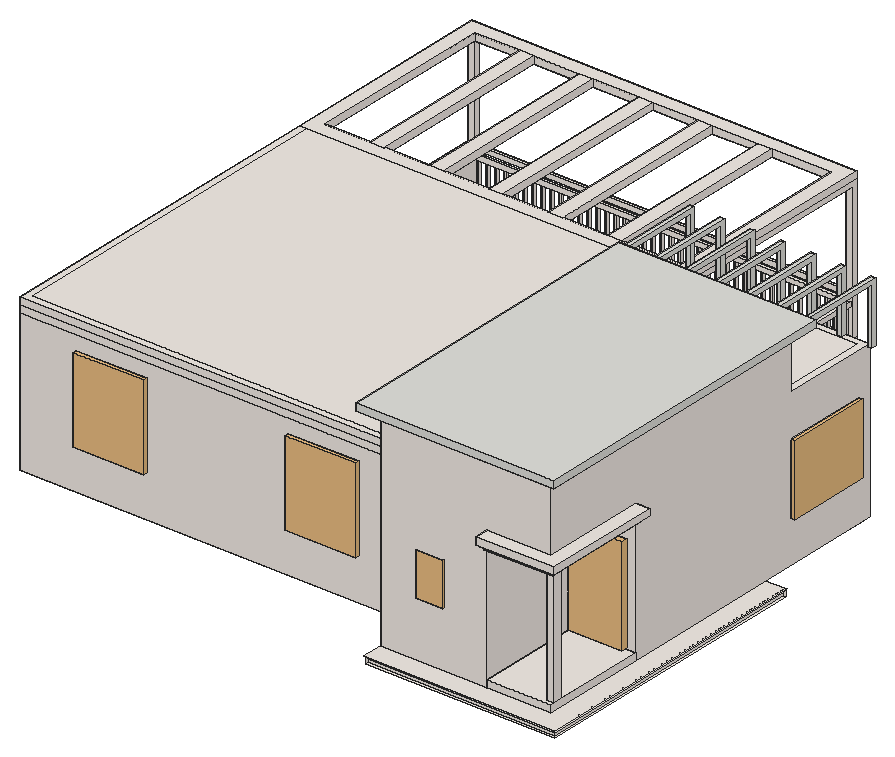
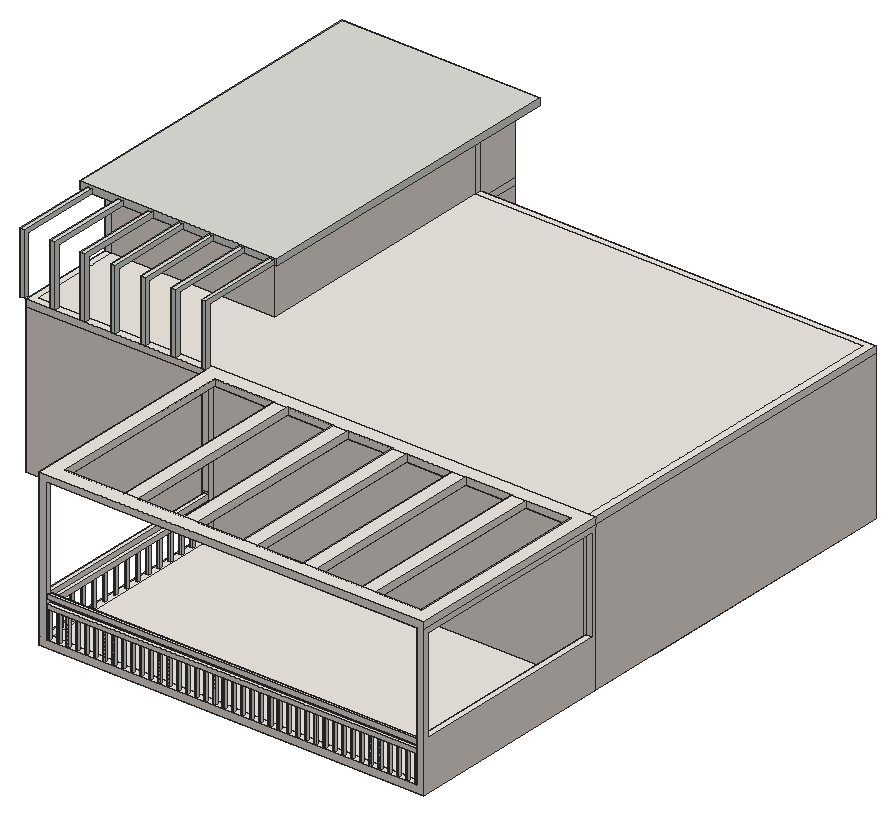
# SketchUp Ruby script. Lengths in inches.
U = 1.inch
M = Sketchup.active_model
def pt(a) = Geom::Point3d.new(a.map { |v| v * U })
def face(e, loops, mat)
  f = e.add_face(loops[0].map { |a| pt(a) })
  loops[1..].each { |l| e.add_face(l.map { |a| pt(a) }).erase! }
  f.material = f.back_material = mat if mat
  f
end
# faces: each face lists its corners as indices into pts; further lists are holes
def faces(e, pts, list, mat = nil) = list.each { |f| face(e, (f[0].is_a?(Array) ? f : [f]).map { |l| l.map { |i| pts[i] } }, mat) }
# xy, xz, yz: faces in a plane at the given z, y or x. An outline is a flat list of corners, or four numbers for a rectangle; further outlines are holes
def ring(l) = l.size == 4 ? [[l[0], l[1]], [l[2], l[1]], [l[2], l[3]], [l[0], l[3]]] : l.each_slice(2).to_a
def flat(e, list, mat, &to3) = list.each { |f| face(e, (f[0].is_a?(Array) ? f : [f]).map { |l| ring(l).map { |u, v| to3.(u, v) } }, mat) }
def xy(e, z, list, mat = nil) = flat(e, list, mat) { |x, y| [x, y, z] }
def xz(e, y, list, mat = nil) = flat(e, list, mat) { |x, z| [x, y, z] }
def yz(e, x, list, mat = nil) = flat(e, list, mat) { |y, z| [x, y, z] }
def lines(e, pts, list) = list.each { |a, b| e.add_line(pt(pts[a]), pt(pts[b])) }
# prism: a flat outline (further loops are holes) pulled along v
def prism(e, loops, v, mat = nil)
  f = face(e, loops, mat); d = Geom::Vector3d.new(v.map { |x| x * U })
  f.pushpull(f.normal.samedirection?(d) ? d.length : -d.length)
end
def box(e, o, s, mat = nil) = prism(e, [[o, [o[0] + s[0], o[1], o[2]], [o[0] + s[0], o[1] + s[1], o[2]], [o[0], o[1] + s[1], o[2]]]], [0, 0, s[2]], mat)
def at(x, y, z, deg = 0) = Geom::Transformation.translation(pt([x, y, z])) * Geom::Transformation.rotation(ORIGIN, Z_AXIS, deg.degrees)
def axes(o, x, y, z) = Geom::Transformation.new([*x, 0, *y, 0, *z, 0, *pt(o).to_a, 1])
def part(name) = M.definitions.add(name)
# library, detail: a bought-in or finely detailed component or shape, given as its bounding box
def library(name, o, s) = part(name).tap { |d| box(d.entities, o, s) }
def detail(e, o, s) = box(e.add_group.entities, o, s)
def put(e, d, t, mat = nil) = e.add_instance(d, t).tap { |i| i.material = mat if mat }
def group(e, t, mat = nil) = e.add_group.tap { |g| g.transformation = t; g.material = mat if mat }.entities
root = M.entities
M.materials.add("D01_Frost_White").color = [242, 235, 229]
c1 = library("porta+4",[0.2,-5.42,1.33],[46.55,4.72,83.21])
c2 = library("mesh-163",[-551.08,-704.17,-20.03],[1929.24,1401.85,86.96])
c3 = part("Group11")
put(c3.entities,c2,at(0,0,0))
xy(root,373,[[349,0,510,0,510,245,508,245,508,2,349,2]],"D01_Frost_White")
xy(root,377,[[349,0,508,2],[508,0,510,245]],"D01_Frost_White")
xy(root,378,[[348,0,510,0,510,246,492,246,492,18,348,18],[348,18,438,18,438,60,18,60,18,54,348,54],[438,18,486,60],[486,18,492,108],[12,54,18,288],
  [18,60,192,288],[192,60,198,288],[198,60,198,288,486,288,486,210,342,210,342,60],[342,60,348,60,348,204,486,204,486,108,492,108,492,288,486,288,486,210,342,210],[348,60,348,204,486,204,486,114,433.5,114,433.5,60],
  [433.5,60,433.5,114,486,114,486,108,438,108,438,60],[438,60,486,108],[12,288,198,294],[198,288,486,294],[486,288,492,294],
  [12,294,18,528],[18,294,18,528,255,528,255,471,333,471,333,351,486,351,486,294],[486,294,492,351],[333,351,492,351,492,357,339,357,339,471,333,471],[255,471,333,471,333,477,261,477,261,528,255,528],
  [333,471,339,477],[261,477,333,528],[333,477,339,528],[12,528,339,534]],"D01_Frost_White")
xy(root,383.99,[[96.4,531.13,98.4,533.13],[104.2,531.13,106.2,533.13],[112,531.13,114,533.13],[119.8,531.13,121.8,533.13],[127.6,531.13,129.6,533.13],
  [135.4,531.13,137.4,533.13],[143.2,531.13,145.2,533.13],[151,531.13,153,533.13],[158.79,531.13,160.79,533.13],[166.59,531.13,168.59,533.13],
  [174.39,531.13,176.39,533.13],[182.19,531.13,184.19,533.13],[189.99,531.13,191.99,533.13],[197.79,531.13,199.79,533.13],[205.59,531.13,207.59,533.13],
  [213.38,531.13,215.38,533.13],[221.18,531.13,223.18,533.13],[228.98,531.13,230.98,533.13],[236.78,531.13,238.78,533.13],[244.58,531.13,246.58,533.13],
  [252.38,531.13,254.38,533.13],[260.18,531.13,262.18,533.13],[267.98,531.13,269.98,533.13],[275.77,531.13,277.77,533.13],[283.57,531.13,285.57,533.13],
  [291.37,531.13,293.37,533.13],[299.17,531.13,301.17,533.13],[306.97,531.13,308.97,533.13],[314.77,531.13,316.77,533.13],[322.57,531.13,324.57,533.13],
  [330.37,531.13,332.37,533.13]],"D01_Frost_White")
xy(root,384,[[438,18,492,18,492,21.03,486,21.03,486,29,492,29,492,108,438,108],[18,60,432,60,432,114,486,114,486,351,18,351],[18,357,333,528],[[333,361,339,530],[334.61,362.99,336.61,364.99],[334.61,374.65,336.61,376.65],[334.61,386.32,336.61,388.32],[334.61,397.98,336.61,399.98],[334.61,409.64,336.61,411.64],[334.61,421.3,336.61,423.3],[334.61,432.97,336.61,434.97],[334.61,444.63,336.61,446.63],[334.61,456.29,336.61,458.29],[334.61,467.95,336.61,469.95],[334.61,479.61,336.61,481.61],[334.61,491.28,336.61,493.28],[334.61,502.9375,336.61,504.9375],[334.61,514.6,336.61,516.6],[334.61,526.26,336.61,528.26]],[[18,528,333,534],[18.42,531.13,20.42,533.13],[26.22,531.13,28.22,533.13],[34.02,531.13,36.02,533.13],[41.8125,531.13,43.8125,533.13],[49.61,531.13,51.61,533.13],[57.41,531.13,59.41,533.13],[73.01,531.13,75.01,533.13],[65.21,531.13,67.21,533.13],[80.81,531.13,82.81,533.13],[88.61,531.13,90.61,533.13]]],"D01_Frost_White")
xy(root,387,[[441,108,471,114]],"D01_Frost_White")
xy(root,407.45,[[[333.5,361,337.5,530],[334.61,362.99,336.61,364.99],[334.61,374.65,336.61,376.65],[334.61,386.32,336.61,388.32],[334.61,397.98,336.61,399.98],[334.61,409.64,336.61,411.64],[334.61,421.3,336.61,423.3],[334.61,432.97,336.61,434.97],[334.61,444.63,336.61,446.63],[334.61,456.29,336.61,458.29],[334.61,467.95,336.61,469.95],[334.61,479.61,336.61,481.61],[334.61,491.28,336.61,493.28],[334.61,502.9375,336.61,504.9375],[334.61,514.6,336.61,516.6],[334.61,526.26,336.61,528.26]],[[18,530.5,333,533.39],[330.37,531.13,332.37,533.13],[322.57,531.13,324.57,533.13],[314.77,531.13,316.77,533.13],[306.97,531.13,308.97,533.13],[299.17,531.13,301.17,533.13],[291.37,531.13,293.37,533.13],[283.57,531.13,285.57,533.13],[275.77,531.13,277.77,533.13],[267.98,531.13,269.98,533.13],[260.18,531.13,262.18,533.13],[252.38,531.13,254.38,533.13],[244.58,531.13,246.58,533.13],[236.78,531.13,238.78,533.13],[228.98,531.13,230.98,533.13],[221.18,531.13,223.18,533.13],[213.38,531.13,215.38,533.13],[205.59,531.13,207.59,533.13],[197.79,531.13,199.79,533.13],[189.99,531.13,191.99,533.13],[182.19,531.13,184.19,533.13],[174.39,531.13,176.39,533.13],[166.59,531.13,168.59,533.13],[158.79,531.13,160.79,533.13],[151,531.13,153,533.13],[143.2,531.13,145.2,533.13],[135.4,531.13,137.4,533.13],[127.6,531.13,129.6,533.13],[119.8,531.13,121.8,533.13],[112,531.13,114,533.13],[104.2,531.13,106.2,533.13],[96.4,531.13,98.4,533.13],[88.61,531.13,90.61,533.13],[80.81,531.13,82.81,533.13],[73.01,531.13,75.01,533.13],[65.21,531.13,67.21,533.13],[57.41,531.13,59.41,533.13],[49.61,531.13,51.61,533.13],[41.8125,531.13,43.8125,533.13],[34.02,531.13,36.02,533.13],[26.22,531.13,28.22,533.13],[18.42,531.13,20.42,533.13]],[18,533.39,333,533.5]],"D01_Frost_White")
xy(root,411.45,[[333.5,361,337.5,530],[18,530.5,333,533.5]],"D01_Frost_White")
xy(root,414.58,[[333.5,361,337.5,530],[18,530.5,333,533.39],[18,533.39,333,533.5]],"D01_Frost_White")
xy(root,416,[[62,54,108,60],[108,54,118,60],[242,54,288,60],[288,54,298,60],[486,275,492,343]],"D01_Frost_White")
xy(root,418.58,[[333.5,361,337.5,530],[18,530.5,333,533.5]],"D01_Frost_White")
xy(root,420,[[12,355,18,530]],"D01_Frost_White")
xy(root,428,[[380,18,400,60]],"D01_Frost_White")
xy(root,460,[[380,18,400,60]],"D01_Frost_White")
xy(root,465,[[441,108,471,114]],"D01_Frost_White")
xy(root,472,[[486,275,492,343]],"D01_Frost_White")
xy(root,484,[[62,54,118,60],[242,54,298,60]],"D01_Frost_White")
xy(root,488,[[[442,10,500,104],[486,21.03,492,29]]],"D01_Frost_White")
xy(root,490,[[[440,8,502,106],[442,10,500,104]]],"D01_Frost_White")
xy(root,492,[[[438,6,504,108],[440,8,502,106]],[486,21.03,492,29]],"D01_Frost_White")
xy(root,498,[[438,6,504,6,504,108,492,108,492,18,438,18]],"D01_Frost_White")
xy(root,500,[[12,355,18,530],[333,361,339,530]],"D01_Frost_White")
xy(root,504,[[18,60,18,351,486,351,486,114,432,114,432,60],[[18,357,333,534],[276.5,363,327,522],[226,363,264.5,522],[24,363,62.5,522],[175.5,363,214,522],[125,363,163.5,522],[74.5,363,113,522]]],"D01_Frost_White")
xy(root,510,[[338.96,353,342.88,357],[364.67,353,368.6,357],[390.38,353,394.31,357],[416.1,353,420.02,357],[441.81,353,445.74,357],
  [467.52,353,471.45,357],[493.23,353,497.16,357]])
xy(root,510,[[354,24,486,267],[12,54,348,54,348,60,18,60,18,351,12,351],[18,60,348,60,348,273,486,273,486,351,18,351],[[486,273,492,273,492,357,339,357,339,534,12,534,12,351,486,351],[24,363,327,522]],[62.5,363,74.5,522],
  [113,363,125,522],[163.5,363,175.5,522],[214,363,226,522],[264.5,363,276.5,522]],"D01_Frost_White")
xy(root,558,[[336,6,336,285,338.96,285,338.96,353,342.88,353,342.88,285,364.67,285,364.67,353,368.6,353,368.6,285,390.38,285,390.38,353,394.31,353,394.31,285,416.1,285,416.1,353,420.02,353,420.02,285,441.81,285,441.81,353,445.74,353,445.74,285,467.52,285,467.52,353,471.45,353,471.45,285,493.23,285,493.23,353,497.16,353,497.16,285,504,285,504,6]])
xy(root,558,[[[348,18,492,273],[354,24,486,267]]],"D01_Frost_White")
xy(root,561.93,[[338.96,285,342.88,357],[364.67,285,368.6,357],[390.38,285,394.31,357],[416.1,285,420.02,357],[441.81,285,445.74,357],
  [467.52,285,471.45,357],[493.23,285,497.16,357]])
xy(root,564,[[336,6,504,285]])
xz(root,2,[[349,373,508,377]],"D01_Frost_White")
xz(root,6,[[336,558,504,564]])
xz(root,6,[[438,492,504,498]],"D01_Frost_White")
xz(root,8,[[440,490,502,492]],"D01_Frost_White")
xz(root,10,[[442,488,500,490]],"D01_Frost_White")
xz(root,18,[[[348,378,438,378,438,498,492,498,492,558,348,558],[378,426,402,462]],[438,378,492,384],[[378,426,402,462],[380,428,400,460]]],"D01_Frost_White")
xz(root,21.03,[[486,384,492,488],[486,488,492,492]],"D01_Frost_White")
xz(root,24,[[354,510,486,558]],"D01_Frost_White")
xz(root,29,[[486,384,492,488],[486,488,492,492]],"D01_Frost_White")
xz(root,54,[[[12,378,348,498],[60,414,120,486],[240,414,300,486]],[[60,414,120,486],[62,416,118,484]],[[240,414,300,486],[242,416,298,484]],[12,498,348,504],[12,504,348,510]],"D01_Frost_White")
xz(root,60,[[[18,384,432,504],[242,416,298,484],[62,416,118,484],[380,428,400,460]]],"D01_Frost_White")
xz(root,104,[[442,488,486,490],[486,488,492,490],[492,488,500,490]],"D01_Frost_White")
xz(root,106,[[440,490,486,492],[486,490,492,492],[492,490,502,492]],"D01_Frost_White")
xz(root,108,[[438,378,492,384],[474,384,492,384,492,492,438,492,438,468,474,468],[[438,384,474,468],[441,387,471,465]],[492,492,504,498]],"D01_Frost_White")
xz(root,114,[[[432,384,486,504],[441,387,471,465]]],"D01_Frost_White")
xz(root,245,[[508,373,510,377]],"D01_Frost_White")
xz(root,267,[[354,510,486,558]],"D01_Frost_White")
xz(root,273,[[348,510,486,558],[486,510,492,558]],"D01_Frost_White")
xz(root,275,[[486,416,492,472]],"D01_Frost_White")
xz(root,285,[[336,558,336,564,504,564,504,558,497.16,558,497.16,561.93,493.23,561.93,493.23,558,471.45,558,471.45,561.93,467.52,561.93,467.52,558,445.74,558,445.74,561.93,441.81,561.93,441.81,558,420.02,558,420.02,561.93,416.1,561.93,416.1,558,394.31,558,394.31,561.93,390.38,561.93,390.38,558,368.6,558,368.6,561.93,364.67,561.93,364.67,558,342.88,558,342.88,561.93,338.96,561.93,338.96,558]])
xz(root,343,[[486,416,492,472]],"D01_Frost_White")
xz(root,351,[[18,384,486,504]],"D01_Frost_White")
xz(root,353,[[338.96,510,342.88,558],[364.67,510,368.6,558],[390.38,510,394.31,558],[416.1,510,420.02,558],[441.81,510,445.74,558],
  [467.52,510,471.45,558],[493.23,510,497.16,558]])
xz(root,355,[[12,420,18,500]],"D01_Frost_White")
xz(root,357,[[338.96,510,342.88,561.93],[364.67,510,368.6,561.93],[390.38,510,394.31,561.93],[416.1,510,420.02,561.93],[441.81,510,445.74,561.93],
  [467.52,510,471.45,561.93],[493.23,510,497.16,561.93]])
xz(root,357,[[339,378,492,504],[18,384,333,504],[339,504,492,510]],"D01_Frost_White")
xz(root,361,[[[333,384,339,420],[333.5,414.58,337.5,418.58],[333.5,407.45,337.5,411.45],[333.5,400.33,337.5,404.33],[333.5,393.2,337.5,397.2],[333.5,386.08,337.5,390.08]],[333.5,386.08,337.5,390.08],[333.5,393.2,337.5,397.2],[333.5,400.33,337.5,404.33],[333,420,339,500]],"D01_Frost_White")
xz(root,362.99,[[334.61,384,336.61,407.45]],"D01_Frost_White")
xz(root,363,[[24,504,62.5,510],[74.5,504,113,510],[125,504,163.5,510],[175.5,504,214,510],[226,504,264.5,510],
  [276.5,504,327,510]],"D01_Frost_White")
xz(root,364.99,[[334.61,384,336.61,407.45]],"D01_Frost_White")
xz(root,374.65,[[334.61,384,336.61,407.45]],"D01_Frost_White")
xz(root,376.65,[[334.61,384,336.61,407.45]],"D01_Frost_White")
xz(root,386.32,[[334.61,384,336.61,407.45]],"D01_Frost_White")
xz(root,388.32,[[334.61,384,336.61,407.45]],"D01_Frost_White")
xz(root,397.98,[[334.61,384,336.61,407.45]],"D01_Frost_White")
xz(root,399.98,[[334.61,384,336.61,407.45]],"D01_Frost_White")
xz(root,409.64,[[334.61,384,336.61,407.45]],"D01_Frost_White")
xz(root,411.64,[[334.61,384,336.61,407.45]],"D01_Frost_White")
xz(root,421.3,[[334.61,384,336.61,407.45]],"D01_Frost_White")
xz(root,423.3,[[334.61,384,336.61,407.45]],"D01_Frost_White")
xz(root,432.97,[[334.61,384,336.61,407.45]],"D01_Frost_White")
xz(root,434.97,[[334.61,384,336.61,407.45]],"D01_Frost_White")
xz(root,444.63,[[334.61,384,336.61,407.45]],"D01_Frost_White")
xz(root,446.63,[[334.61,384,336.61,407.45]],"D01_Frost_White")
xz(root,456.29,[[334.61,384,336.61,407.45]],"D01_Frost_White")
xz(root,458.29,[[334.61,384,336.61,407.45]],"D01_Frost_White")
xz(root,467.95,[[334.61,384,336.61,407.45]],"D01_Frost_White")
xz(root,469.95,[[334.61,384,336.61,407.45]],"D01_Frost_White")
xz(root,479.61,[[334.61,384,336.61,407.45]],"D01_Frost_White")
xz(root,481.61,[[334.61,384,336.61,407.45]],"D01_Frost_White")
xz(root,491.28,[[334.61,384,336.61,407.45]],"D01_Frost_White")
xz(root,493.28,[[334.61,384,336.61,407.45]],"D01_Frost_White")
xz(root,502.9375,[[334.61,384,336.61,407.45]],"D01_Frost_White")
xz(root,504.9375,[[334.61,384,336.61,407.45]],"D01_Frost_White")
xz(root,514.6,[[334.61,384,336.61,407.45]],"D01_Frost_White")
xz(root,516.6,[[334.61,384,336.61,407.45]],"D01_Frost_White")
xz(root,522,[[24,504,62.5,510],[74.5,504,113,510],[125,504,163.5,510],[175.5,504,214,510],[226,504,264.5,510],
  [276.5,504,327,510]],"D01_Frost_White")
xz(root,526.26,[[334.61,384,336.61,407.45]],"D01_Frost_White")
xz(root,528.26,[[334.61,384,336.61,407.45]],"D01_Frost_White")
xz(root,530,[[[333,384,339,384,339,500,333,500,333,418.58,337.5,418.58,337.5,414.58,333,414.58],[333.5,407.45,337.5,411.45]],[333,414.58,333.5,418.58],[12,420,18,500]],"D01_Frost_White")
xz(root,530.5,[[18,407.45,333,411.45],[18,414.58,333,418.58]],"D01_Frost_White")
xz(root,531.13,[[96.4,383.99,98.4,407.45],[104.2,383.99,106.2,407.45],[112,383.99,114,407.45],[119.8,383.99,121.8,407.45],[127.6,383.99,129.6,407.45],
  [135.4,383.99,137.4,407.45],[143.2,383.99,145.2,407.45],[151,383.99,153,407.45],[158.79,383.99,160.79,407.45],[166.59,383.99,168.59,407.45],
  [174.39,383.99,176.39,407.45],[182.19,383.99,184.19,407.45],[189.99,383.99,191.99,407.45],[197.79,383.99,199.79,407.45],[205.59,383.99,207.59,407.45],
  [213.38,383.99,215.38,407.45],[221.18,383.99,223.18,407.45],[228.98,383.99,230.98,407.45],[236.78,383.99,238.78,407.45],[244.58,383.99,246.58,407.45],
  [252.38,383.99,254.38,407.45],[260.18,383.99,262.18,407.45],[267.98,383.99,269.98,407.45],[275.77,383.99,277.77,407.45],[283.57,383.99,285.57,407.45],
  [291.37,383.99,293.37,407.45],[299.17,383.99,301.17,407.45],[306.97,383.99,308.97,407.45],[314.77,383.99,316.77,407.45],[322.57,383.99,324.57,407.45],
  [330.37,383.99,332.37,407.45],[18.42,384,20.42,407.45],[26.22,384,28.22,407.45],[34.02,384,36.02,407.45],[41.8125,384,43.8125,407.45],
  [49.61,384,51.61,407.45],[57.41,384,59.41,407.45],[65.21,384,67.21,407.45],[73.01,384,75.01,407.45],[80.81,384,82.81,407.45],
  [88.61,384,90.61,407.45]],"D01_Frost_White")
xz(root,533.13,[[96.4,383.99,97.3,407.45],[97.3,383.99,98.4,407.45],[104.2,383.99,105.1,407.45],[105.1,383.99,106.2,407.45],[112,383.99,112.9,407.45],
  [112.9,383.99,114,407.45],[119.8,383.99,120.7,407.45],[120.7,383.99,121.8,407.45],[127.6,383.99,128.49,407.45],[128.49,383.99,129.6,407.45],
  [135.4,383.99,136.29,407.45],[136.29,383.99,137.4,407.45],[143.2,383.99,144.09,407.45],[144.09,383.99,145.2,407.45],[151,383.99,151.89,407.45],
  [151.89,383.99,153,407.45],[158.79,383.99,159.6875,407.45],[159.6875,383.99,160.79,407.45],[166.59,383.99,167.49,407.45],[167.49,383.99,168.59,407.45],
  [174.39,383.99,175.29,407.45],[175.29,383.99,176.39,407.45],[182.19,383.99,183.08,407.45],[183.08,383.99,184.19,407.45],[189.99,383.99,190.88,407.45],
  [190.88,383.99,191.99,407.45],[197.79,383.99,198.68,407.45],[198.68,383.99,199.79,407.45],[205.59,383.99,206.48,407.45],[206.48,383.99,207.59,407.45],
  [213.38,383.99,214.28,407.45],[214.28,383.99,215.38,407.45],[221.18,383.99,222.08,407.45],[222.08,383.99,223.18,407.45],[228.98,383.99,229.875,407.45],
  [229.875,383.99,230.98,407.45],[236.78,383.99,237.68,407.45],[237.68,383.99,238.78,407.45],[244.58,383.99,245.47,407.45],[245.47,383.99,246.58,407.45],
  [252.38,383.99,253.27,407.45],[253.27,383.99,254.38,407.45],[260.18,383.99,261.07,407.45],[261.07,383.99,262.18,407.45],[267.98,383.99,268.87,407.45],
  [268.87,383.99,269.98,407.45],[275.77,383.99,276.67,407.45],[276.67,383.99,277.77,407.45],[283.57,383.99,284.47,407.45],[284.47,383.99,285.57,407.45],
  [291.37,383.99,292.27,407.45],[292.27,383.99,293.37,407.45],[299.17,383.99,300.06,407.45],[300.06,383.99,301.17,407.45],[306.97,383.99,307.86,407.45],
  [307.86,383.99,308.97,407.45],[314.77,383.99,315.66,407.45],[315.66,383.99,316.77,407.45],[322.57,383.99,323.46,407.45],[323.46,383.99,324.57,407.45],
  [330.37,383.99,331.26,407.45],[331.26,383.99,332.37,407.45],[18.42,384,19.3125,407.45],[19.3125,384,20.42,407.45],[26.22,384,27.11,407.45],
  [27.11,384,28.22,407.45],[34.02,384,34.91,407.45],[34.91,384,36.02,407.45],[41.8125,384,42.71,407.45],[42.71,384,43.8125,407.45],
  [49.61,384,50.51,407.45],[50.51,384,51.61,407.45],[57.41,384,58.31,407.45],[58.31,384,59.41,407.45],[65.21,384,66.1,407.45],
  [66.1,384,67.21,407.45],[73.01,384,73.9,407.45],[73.9,384,75.01,407.45],[80.81,384,81.7,407.45],[81.7,384,82.81,407.45],
  [88.61,384,89.5,407.45],[89.5,384,90.61,407.45]],"D01_Frost_White")
xz(root,533.5,[[18,407.45,333,411.45],[18,414.58,333,418.58]],"D01_Frost_White")
xz(root,534,[[12,378,12,510,339,510,339,384,333,384,333,504,18,504,18,384,339,384,339,378]],"D01_Frost_White")
yz(root,12,[[54,378,351,504],[[351,378,534,504],[355,420,530,500]],[54,504,351,510],[351,504,534,510]],"D01_Frost_White")
yz(root,18,[[60,384,351,504],[355,384,357,420],[[357,384,534,384,534,504,357,504,357,500,530,500,530,420,357,420],[530.5,414.58,533.5,418.58],[530.5,407.45,533.5,411.45]],[355,420,357,500]],"D01_Frost_White")
yz(root,18.42,[[531.13,384,533.13,407.45]],"D01_Frost_White")
yz(root,20.42,[[531.13,384,533.13,407.45]],"D01_Frost_White")
yz(root,24,[[363,504,522,510]],"D01_Frost_White")
yz(root,26.22,[[531.13,384,533.13,407.45]],"D01_Frost_White")
yz(root,28.22,[[531.13,384,533.13,407.45]],"D01_Frost_White")
yz(root,34.02,[[531.13,384,533.13,407.45]],"D01_Frost_White")
yz(root,36.02,[[531.13,384,533.13,407.45]],"D01_Frost_White")
yz(root,41.8125,[[531.13,384,533.13,407.45]],"D01_Frost_White")
yz(root,43.8125,[[531.13,384,533.13,407.45]],"D01_Frost_White")
yz(root,49.61,[[531.13,384,533.13,407.45]],"D01_Frost_White")
yz(root,51.61,[[531.13,384,533.13,407.45]],"D01_Frost_White")
yz(root,57.41,[[531.13,384,533.13,407.45]],"D01_Frost_White")
yz(root,59.41,[[531.13,384,533.13,407.45]],"D01_Frost_White")
yz(root,62,[[54,416,60,474],[54,474,60,484]],"D01_Frost_White")
yz(root,62.5,[[363,504,522,510]],"D01_Frost_White")
yz(root,65.21,[[531.13,384,533.13,407.45]],"D01_Frost_White")
yz(root,67.21,[[531.13,384,533.13,407.45]],"D01_Frost_White")
yz(root,73.01,[[531.13,384,533.13,407.45]],"D01_Frost_White")
yz(root,74.5,[[363,504,522,510]],"D01_Frost_White")
yz(root,75.01,[[531.13,384,533.13,407.45]],"D01_Frost_White")
yz(root,80.81,[[531.13,384,533.13,407.45]],"D01_Frost_White")
yz(root,82.81,[[531.13,384,533.13,407.45]],"D01_Frost_White")
yz(root,88.61,[[531.13,384,533.13,407.45]],"D01_Frost_White")
yz(root,90.61,[[531.13,384,533.13,407.45]],"D01_Frost_White")
yz(root,96.4,[[531.13,383.99,533.13,407.45]],"D01_Frost_White")
yz(root,98.4,[[531.13,383.99,533.13,407.45]],"D01_Frost_White")
yz(root,104.2,[[531.13,383.99,533.13,407.45]],"D01_Frost_White")
yz(root,106.2,[[531.13,383.99,533.13,407.45]],"D01_Frost_White")
yz(root,112,[[531.13,383.99,533.13,407.45]],"D01_Frost_White")
yz(root,113,[[363,504,522,510]],"D01_Frost_White")
yz(root,114,[[531.13,383.99,533.13,407.45]],"D01_Frost_White")
yz(root,118,[[54,416,60,484]],"D01_Frost_White")
yz(root,119.8,[[531.13,383.99,533.13,407.45]],"D01_Frost_White")
yz(root,121.8,[[531.13,383.99,533.13,407.45]],"D01_Frost_White")
yz(root,125,[[363,504,522,510]],"D01_Frost_White")
yz(root,127.6,[[531.13,383.99,533.13,407.45]],"D01_Frost_White")
yz(root,129.6,[[531.13,383.99,533.13,407.45]],"D01_Frost_White")
yz(root,135.4,[[531.13,383.99,533.13,407.45]],"D01_Frost_White")
yz(root,137.4,[[531.13,383.99,533.13,407.45]],"D01_Frost_White")
yz(root,143.2,[[531.13,383.99,533.13,407.45]],"D01_Frost_White")
yz(root,145.2,[[531.13,383.99,533.13,407.45]],"D01_Frost_White")
yz(root,151,[[531.13,383.99,533.13,407.45]],"D01_Frost_White")
yz(root,153,[[531.13,383.99,533.13,407.45]],"D01_Frost_White")
yz(root,158.79,[[531.13,383.99,533.13,407.45]],"D01_Frost_White")
yz(root,160.79,[[531.13,383.99,533.13,407.45]],"D01_Frost_White")
yz(root,163.5,[[363,504,522,510]],"D01_Frost_White")
yz(root,166.59,[[531.13,383.99,533.13,407.45]],"D01_Frost_White")
yz(root,168.59,[[531.13,383.99,533.13,407.45]],"D01_Frost_White")
yz(root,174.39,[[531.13,383.99,533.13,407.45]],"D01_Frost_White")
yz(root,175.5,[[363,504,522,510]],"D01_Frost_White")
yz(root,176.39,[[531.13,383.99,533.13,407.45]],"D01_Frost_White")
yz(root,182.19,[[531.13,383.99,533.13,407.45]],"D01_Frost_White")
yz(root,184.19,[[531.13,383.99,533.13,407.45]],"D01_Frost_White")
yz(root,189.99,[[531.13,383.99,533.13,407.45]],"D01_Frost_White")
yz(root,191.99,[[531.13,383.99,533.13,407.45]],"D01_Frost_White")
yz(root,197.79,[[531.13,383.99,533.13,407.45]],"D01_Frost_White")
yz(root,199.79,[[531.13,383.99,533.13,407.45]],"D01_Frost_White")
yz(root,205.59,[[531.13,383.99,533.13,407.45]],"D01_Frost_White")
yz(root,207.59,[[531.13,383.99,533.13,407.45]],"D01_Frost_White")
yz(root,213.38,[[531.13,383.99,533.13,407.45]],"D01_Frost_White")
yz(root,214,[[363,504,522,510]],"D01_Frost_White")
yz(root,215.38,[[531.13,383.99,533.13,407.45]],"D01_Frost_White")
yz(root,221.18,[[531.13,383.99,533.13,407.45]],"D01_Frost_White")
yz(root,223.18,[[531.13,383.99,533.13,407.45]],"D01_Frost_White")
yz(root,226,[[363,504,522,510]],"D01_Frost_White")
yz(root,228.98,[[531.13,383.99,533.13,407.45]],"D01_Frost_White")
yz(root,230.98,[[531.13,383.99,533.13,407.45]],"D01_Frost_White")
yz(root,236.78,[[531.13,383.99,533.13,407.45]],"D01_Frost_White")
yz(root,238.78,[[531.13,383.99,533.13,407.45]],"D01_Frost_White")
yz(root,242,[[54,416,60,474],[54,474,60,484]],"D01_Frost_White")
yz(root,244.58,[[531.13,383.99,533.13,407.45]],"D01_Frost_White")
yz(root,246.58,[[531.13,383.99,533.13,407.45]],"D01_Frost_White")
yz(root,252.38,[[531.13,383.99,533.13,407.45]],"D01_Frost_White")
yz(root,254.38,[[531.13,383.99,533.13,407.45]],"D01_Frost_White")
yz(root,260.18,[[531.13,383.99,533.13,407.45]],"D01_Frost_White")
yz(root,262.18,[[531.13,383.99,533.13,407.45]],"D01_Frost_White")
yz(root,264.5,[[363,504,522,510]],"D01_Frost_White")
yz(root,267.98,[[531.13,383.99,533.13,407.45]],"D01_Frost_White")
yz(root,269.98,[[531.13,383.99,533.13,407.45]],"D01_Frost_White")
yz(root,275.77,[[531.13,383.99,533.13,407.45]],"D01_Frost_White")
yz(root,276.5,[[363,504,522,510]],"D01_Frost_White")
yz(root,277.77,[[531.13,383.99,533.13,407.45]],"D01_Frost_White")
yz(root,283.57,[[531.13,383.99,533.13,407.45]],"D01_Frost_White")
yz(root,285.57,[[531.13,383.99,533.13,407.45]],"D01_Frost_White")
yz(root,291.37,[[531.13,383.99,533.13,407.45]],"D01_Frost_White")
yz(root,293.37,[[531.13,383.99,533.13,407.45]],"D01_Frost_White")
yz(root,298,[[54,416,60,484]],"D01_Frost_White")
yz(root,299.17,[[531.13,383.99,533.13,407.45]],"D01_Frost_White")
yz(root,301.17,[[531.13,383.99,533.13,407.45]],"D01_Frost_White")
yz(root,306.97,[[531.13,383.99,533.13,407.45]],"D01_Frost_White")
yz(root,308.97,[[531.13,383.99,533.13,407.45]],"D01_Frost_White")
yz(root,314.77,[[531.13,383.99,533.13,407.45]],"D01_Frost_White")
yz(root,316.77,[[531.13,383.99,533.13,407.45]],"D01_Frost_White")
yz(root,322.57,[[531.13,383.99,533.13,407.45]],"D01_Frost_White")
yz(root,324.57,[[531.13,383.99,533.13,407.45]],"D01_Frost_White")
yz(root,327,[[363,504,522,510]],"D01_Frost_White")
yz(root,330.37,[[531.13,383.99,533.13,407.45]],"D01_Frost_White")
yz(root,332.37,[[531.13,383.99,533.13,407.45]],"D01_Frost_White")
yz(root,333,[[[357,384,357,504,534,504,534,384,530,384,530,500,361,500,361,384],[530.5,414.58,533.5,418.58],[530.5,407.45,533.5,411.45]]],"D01_Frost_White")
yz(root,333.5,[[361,407.45,530,411.45],[361,414.58,530,418.58]],"D01_Frost_White")
yz(root,334.61,[[362.99,384,364.99,407.45],[374.65,384,376.65,407.45],[386.32,384,388.32,407.45],[397.98,384,399.98,407.45],[409.64,384,411.64,407.45],
  [421.3,384,423.3,407.45],[432.97,384,434.97,407.45],[444.63,384,446.63,407.45],[456.29,384,458.29,407.45],[467.95,384,469.95,407.45],
  [479.61,384,481.61,407.45],[491.28,384,493.28,407.45],[502.9375,384,504.9375,407.45],[514.6,384,516.6,407.45],[526.26,384,528.26,407.45]],"D01_Frost_White")
yz(root,336,[[6,558,285,564]])
yz(root,336.61,[[362.99,384,364.99,407.45],[374.65,384,376.65,407.45],[386.32,384,388.32,407.45],[397.98,384,399.98,407.45],[409.64,384,411.64,407.45],
  [421.3,384,423.3,407.45],[432.97,384,434.97,407.45],[444.63,384,446.63,407.45],[456.29,384,458.29,407.45],[467.95,384,469.95,407.45],
  [479.61,384,481.61,407.45],[491.28,384,493.28,407.45],[502.9375,384,504.9375,407.45],[514.6,384,516.6,407.45],[526.26,384,528.26,407.45]],"D01_Frost_White")
yz(root,337.5,[[361,407.45,530,411.45],[361,414.58,530,418.58]],"D01_Frost_White")
yz(root,338.96,[[353,510,353,558,285,558,285,561.93,357,561.93,357,510]])
yz(root,339,[[357,378,534,384],[357,384,361,384,361,500,530,500,530,384,534,384,534,504,357,504],[357,504,534,510]],"D01_Frost_White")
yz(root,342.88,[[353,510,357,510,357,561.93,285,561.93,285,558,353,558]])
yz(root,348,[[18,378,54,498],[18,498,54,504],[18,504,54,558],[54,510,60,558],[60,510,273,558]],"D01_Frost_White")
yz(root,349,[[0,373,2,377]],"D01_Frost_White")
yz(root,354,[[24,510,267,558]],"D01_Frost_White")
yz(root,364.67,[[353,510,353,558,285,558,285,561.93,357,561.93,357,510]])
yz(root,368.6,[[353,510,357,510,357,561.93,285,561.93,285,558,353,558]])
yz(root,380,[[18,428,60,460]],"D01_Frost_White")
yz(root,390.38,[[353,510,353,558,285,558,285,561.93,357,561.93,357,510]])
yz(root,394.31,[[353,510,357,510,357,561.93,285,561.93,285,558,353,558]])
yz(root,400,[[18,428,60,460]],"D01_Frost_White")
yz(root,416.1,[[353,510,353,558,285,558,285,561.93,357,561.93,357,510]])
yz(root,420.02,[[353,510,357,510,357,561.93,285,561.93,285,558,353,558]])
yz(root,432,[[60,384,114,492],[60,492,114,504]],"D01_Frost_White")
yz(root,438,[[18,378,108,384],[18,384,108,492],[6,492,18,498]],"D01_Frost_White")
yz(root,440,[[8,490,18,492],[18,490,106,492]],"D01_Frost_White")
yz(root,441,[[108,387,114,465]],"D01_Frost_White")
yz(root,441.81,[[353,510,353,558,285,558,285,561.93,357,561.93,357,510]])
yz(root,442,[[10,488,18,490],[18,488,104,490]],"D01_Frost_White")
yz(root,445.74,[[353,510,357,510,357,561.93,285,561.93,285,558,353,558]])
yz(root,467.52,[[353,510,353,558,285,558,285,561.93,357,561.93,357,510]])
yz(root,471,[[108,387,114,465]],"D01_Frost_White")
yz(root,471.45,[[353,510,357,510,357,561.93,285,561.93,285,558,353,558]])
yz(root,486,[[21.03,384,29,488],[[114,384,351,504],[275,416,343,472]],[21.03,488,29,492],[24,510,267,558]],"D01_Frost_White")
yz(root,492,[[18,378,108,384],[[108,378,357,378,357,510,273,510,273,558,18,558,18,498,108,498],[273,414,345,474]],[21.03,384,29,488],[[273,414,345,474],[275,416,343,472]],[21.03,488,29,492]],"D01_Frost_White")
yz(root,493.23,[[353,510,353,558,285,558,285,561.93,357,561.93,357,510]])
yz(root,497.16,[[353,510,357,510,357,561.93,285,561.93,285,558,353,558]])
yz(root,500,[[10,488,104,490]],"D01_Frost_White")
yz(root,502,[[8,490,106,492]],"D01_Frost_White")
yz(root,504,[[6,558,285,564]])
yz(root,504,[[6,492,108,498]],"D01_Frost_White")
yz(root,508,[[2,373,245,377]],"D01_Frost_White")
p = [[192,60,378],[18,60,378],[18,288,378],[192,288,378],[486,108,384],[486,114,384],
  [486,108,504],[486,114,504],[492,108,504],[432,60,504],[432,18,504],[438,60,504],
  [438,18,504],[486,60,504],[486,18,504],[18,60,504],[12,60,504],[486,351,504],
  [486,357,504],[18,351,504],[18,357,504],[486,108,492],[331.26,531.11,407.45],[332.37,531.11,407.45]]
lines(root,p,[[0,1],[1,2],[2,3],[3,0],[4,5],[6,7],[6,8],[9,10],[11,12],[13,14],[15,16],[17,18],
  [19,20],[6,21],[22,23]])
put(root,c1,at(437.8,108.7,383.46))
put(root,c3,axes([494.63,324.55,444.14],[0,-0.0374,0],[0,0,0.0428],[-0.03937,0,0]))
put(root,c3,axes([77.14,53.21,450.29],[0.0311,0,0],[0,0,0.05118],[0,-0.03937,0]))
put(root,c3,axes([257.14,53.21,450.29],[0.0311,0,0],[0,0,0.05118],[0,-0.03937,0]))
put(root,c3,axes([384.73,17.76,444.03],[0.0122,0,0],[0,0,0.02575],[0,-0.0122,0]))
